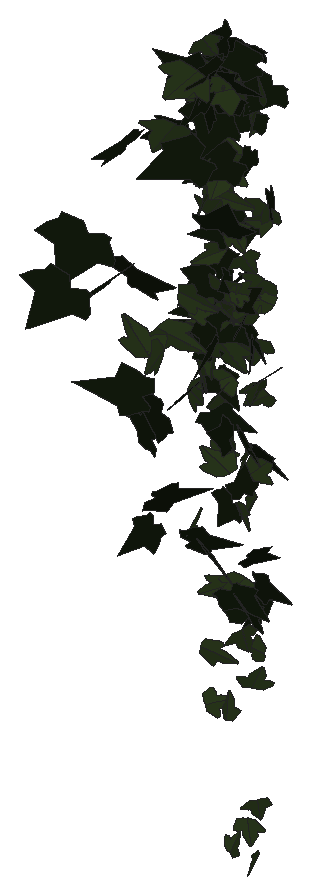
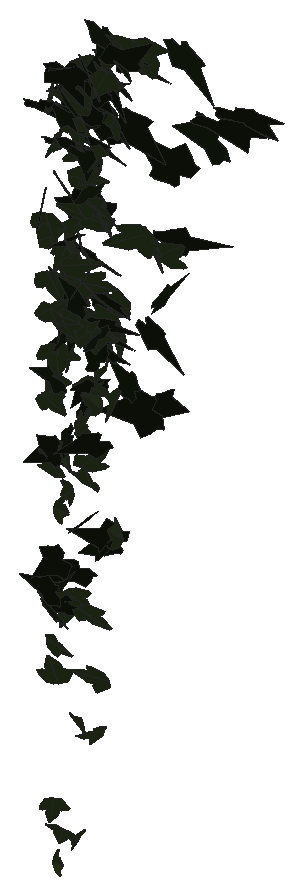
# SketchUp Ruby script. Lengths in inches.
U = 1.inch
M = Sketchup.active_model
def pt(a) = Geom::Point3d.new(a.map { |v| v * U })
def face(e, loops, mat)
  f = e.add_face(loops[0].map { |a| pt(a) })
  loops[1..].each { |l| e.add_face(l.map { |a| pt(a) }).erase! }
  f.material = f.back_material = mat if mat
  f
end
# faces: each face lists its corners as indices into pts; further lists are holes
def faces(e, pts, list, mat = nil) = list.each { |f| face(e, (f[0].is_a?(Array) ? f : [f]).map { |l| l.map { |i| pts[i] } }, mat) }
# xy, xz, yz: faces in a plane at the given z, y or x. An outline is a flat list of corners, or four numbers for a rectangle; further outlines are holes
def ring(l) = l.size == 4 ? [[l[0], l[1]], [l[2], l[1]], [l[2], l[3]], [l[0], l[3]]] : l.each_slice(2).to_a
def flat(e, list, mat, &to3) = list.each { |f| face(e, (f[0].is_a?(Array) ? f : [f]).map { |l| ring(l).map { |u, v| to3.(u, v) } }, mat) }
def xy(e, z, list, mat = nil) = flat(e, list, mat) { |x, y| [x, y, z] }
def xz(e, y, list, mat = nil) = flat(e, list, mat) { |x, z| [x, y, z] }
def yz(e, x, list, mat = nil) = flat(e, list, mat) { |y, z| [x, y, z] }
def lines(e, pts, list) = list.each { |a, b| e.add_line(pt(pts[a]), pt(pts[b])) }
# prism: a flat outline (further loops are holes) pulled along v
def prism(e, loops, v, mat = nil)
  f = face(e, loops, mat); d = Geom::Vector3d.new(v.map { |x| x * U })
  f.pushpull(f.normal.samedirection?(d) ? d.length : -d.length)
end
def box(e, o, s, mat = nil) = prism(e, [[o, [o[0] + s[0], o[1], o[2]], [o[0] + s[0], o[1] + s[1], o[2]], [o[0], o[1] + s[1], o[2]]]], [0, 0, s[2]], mat)
def at(x, y, z, deg = 0) = Geom::Transformation.translation(pt([x, y, z])) * Geom::Transformation.rotation(ORIGIN, Z_AXIS, deg.degrees)
def axes(o, x, y, z) = Geom::Transformation.new([*x, 0, *y, 0, *z, 0, *pt(o).to_a, 1])
def part(name) = M.definitions.add(name)
# library, detail: a bought-in or finely detailed component or shape, given as its bounding box
def library(name, o, s) = part(name).tap { |d| box(d.entities, o, s) }
def detail(e, o, s) = box(e.add_group.entities, o, s)
def put(e, d, t, mat = nil) = e.add_instance(d, t).tap { |i| i.material = mat if mat }
def group(e, t, mat = nil) = e.add_group.tap { |g| g.transformation = t; g.material = mat if mat }.entities
root = M.entities
M.materials.add("1026 AP 7946 SUNNY SIDE UP").color = [254, 231, 186]
M.materials.add("efeu1").color = [18, 25, 13]
M.materials.add("efeu2").color = [43, 57, 29]
c1 = part("ivyleaf_9")
p = [[1.54,2.16,1.25],[1.36,2.04,1.19],[-0.21,0.99,0.68],[-0.71,1.11,0.82],[-0.85,0.86,0.67],[-0.8,0.17,0.21],
  [-0.9,-0.01,0.1],[-0.67,-0.16,-0.02],[-0.08,-0.08,-0.05],[-0.03,-0.6,-0.4],[0.65,-0.88,-0.66],[0.83,-0.6,-0.49],
  [1.29,-0.42,-0.43],[1.8125,-0.07,-0.26],[1.21,0.44,0.15]]
faces(c1.entities,p,[[0,1,2,3,4,5,6,7,8,9,10,11,12,13,14]],"efeu1")
c2 = part("ivyleaf_10")
p = [[0,0.5,-0.03],[-0.0625,2.02,-0.43],[-0.19,2.01,-0.46],[-0.54,1.05,-0.29],[-0.52,0.625,-0.18],[-0.83,0.76,-0.28],
  [-1.16,0.64,-0.33],[-1.15,0.33,-0.24],[-0.77,-0.39,0.02],[-0.3,-0.51,0.16],[0.04,-0.48,0.23],[-0.02,2.01,-0.4375],
  [-0.06,2.01,-0.43],[0.04,-0.49,0.23],[0.67,-0.49,0.14],[1.38,0.36,-0.2],[1.375,0.51,-0.24],[0.81,0.65,-0.19],
  [0.62,0.59,-0.15],[0.6,1.09,-0.28],[0.5,1.23,-0.31]]
faces(c2.entities,p,[[0,1,2,3,4,5,6,7,8,9,10],[11,12,0,13,14,15,16,17,18,19,20]],"efeu2")
put(root,c1,axes([97.74,206.36,264.18],[-0.57261,-0.15899,0.00661],[0.01155,-0.03369,-0.3981],[0.27002,-0.33573,0.03104]),"1026 AP 7946 SUNNY SIDE UP")
put(root,c1,axes([97.83,206.99,263.79],[-0.11865,0.31649,-0.13339],[-0.03463,0.12729,0.34869],[0.57896,0.07247,-0.00648]),"1026 AP 7946 SUNNY SIDE UP")
put(root,c1,axes([97.2,207.625,264.69],[-0.57225,-0.19595,-0.07876],[0.1339,0.00504,-0.41571],[0.32748,-0.34446,0.03235]),"1026 AP 7946 SUNNY SIDE UP")
put(root,c1,axes([98.54,207.72,261.34],[-0.28709,-0.00794,0.3068],[-0.47432,-0.07037,-0.17955],[0.10962,-0.32532,0.02659]),"1026 AP 7946 SUNNY SIDE UP")
put(root,c1,axes([98.41,208.22,260.1],[0.00994,-0.29617,0.10479],[0.00181,0.10178,0.31854],[-0.53159,-0.00519,0.00305]),"1026 AP 7946 SUNNY SIDE UP")
put(root,c1,axes([97.77,208.36,263.6],[0.05912,-0.09662,0.33615],[0.41432,-0.20559,-0.09919],[0.37633,0.24152,0.0564]),"1026 AP 7946 SUNNY SIDE UP")
put(root,c1,axes([98.23,208.49,257.8],[-0.01657,-0.03364,-0.32985],[0.19296,-0.2867,0.0257],[-0.48867,-0.11207,0.02133]),"1026 AP 7946 SUNNY SIDE UP")
put(root,c1,axes([97.62,208.38,266.64],[-0.23235,0.33578,-0.00813],[-0.01483,-0.01648,-0.38812],[-0.57017,-0.1364,0.01341]),"1026 AP 7946 SUNNY SIDE UP")
put(root,c2,axes([98.32,208.6,261.89],[0.27853,-0.2642,-0.07494],[-0.07251,0.05179,-0.3321],[0.45679,0.16932,-0.00702]),"1026 AP 7946 SUNNY SIDE UP")
put(root,c2,axes([97.84,208.8,261.74],[0.42097,0.06657,0.18504],[-0.29585,-0.00962,0.2729],[0.10235,-0.30163,0.02772]),"1026 AP 7946 SUNNY SIDE UP")
put(root,c1,axes([98.88,209.1875,266.44],[-0.59553,-0.0337,0.08502],[-0.12333,-0.06727,-0.37301],[0.08025,-0.35345,0.05773]),"1026 AP 7946 SUNNY SIDE UP")
put(root,c2,axes([98.22,209.02,262.17],[-0.23906,-0.09754,-0.28056],[0.42891,0.07804,-0.17622],[0.19861,-0.28593,0.04286]),"1026 AP 7946 SUNNY SIDE UP")
put(root,c2,axes([98.18,209.22,266.87],[-0.36364,-0.18696,0.13786],[-0.13468,-0.10778,-0.30458],[0.36358,-0.22691,0.02506]),"1026 AP 7946 SUNNY SIDE UP")
put(root,c1,axes([97.92,209.15,260.09],[0.02255,-0.02389,-0.34779],[-0.55102,-0.02407,-0.01266],[-0.03928,0.32393,-0.02202]),"1026 AP 7946 SUNNY SIDE UP")
put(root,c1,axes([97.91,209.13,258.08],[0.04211,0.20914,-0.26445],[-0.00016,0.25047,0.22804],[0.55297,-0.01585,0.0202]),"1026 AP 7946 SUNNY SIDE UP")
put(root,c2,axes([97.86,210.24,267.56],[0.52572,-0.05732,-0.1389],[-0.22518,-0.01183,-0.33548],[0.08194,0.33528,-0.03076]),"1026 AP 7946 SUNNY SIDE UP")
put(root,c1,axes([98.32,210.45,261.27],[-0.2559,0.10294,-0.21454],[0.25125,-0.13866,-0.19608],[-0.29101,-0.21023,0.01936]),"1026 AP 7946 SUNNY SIDE UP")
put(root,c1,axes([98.07,210.53,267.0625],[-0.40271,0.1267,-0.20041],[0.24447,-0.1275,-0.28704],[-0.29877,-0.27511,0.03526]),"1026 AP 7946 SUNNY SIDE UP")
put(root,c1,axes([98.24,210.32,267.7],[-0.19473,0.30654,0.05328],[-0.06802,0.03373,-0.34887],[-0.52171,-0.11882,0.02559]),"1026 AP 7946 SUNNY SIDE UP")
put(root,c1,axes([98.19,210.68,266.55],[-0.27394,-0.27734,0.04395],[0.01113,-0.05522,-0.34245],[0.47673,-0.15808,0.03325]),"1026 AP 7946 SUNNY SIDE UP")
put(root,c1,axes([97.57,210.64,267.34],[0.06166,0.02742,0.27711],[-0.42307,-0.07047,0.04451],[0.12535,-0.25133,0.01393]),"1026 AP 7946 SUNNY SIDE UP")
put(root,c1,axes([97.51,210.6,265.94],[0.0325,0.11967,-0.31584],[-0.40785,-0.19071,-0.10165],[-0.35832,0.22794,0.08705]),"1026 AP 7946 SUNNY SIDE UP")
put(root,c1,axes([97.23,210.5625,259.46],[0.08556,0.22977,0.0797],[-0.03764,-0.06826,0.25078],[0.40672,-0.05465,0.00644]),"1026 AP 7946 SUNNY SIDE UP")
put(root,c1,axes([98.05,210.52,266.88],[0.09166,-0.03664,-0.34822],[-0.55011,0.03688,-0.06161],[0.07227,0.32717,-0.02737]),"1026 AP 7946 SUNNY SIDE UP")
put(root,c1,axes([98.15,210.59,266.2],[-0.2466,0.28893,0.03803],[-0.05451,0.01933,-0.34529],[-0.4904,-0.14744,0.01926]),"1026 AP 7946 SUNNY SIDE UP")
put(root,c2,axes([98.3,210.78,267.125],[0.3436,-0.01208,-0.24927],[-0.39361,-0.04066,-0.21425],[-0.03877,0.30571,-0.034]),"1026 AP 7946 SUNNY SIDE UP")
put(root,c2,axes([97.6875,210.79,260.38],[-0.14335,0.16252,-0.14526],[0.08778,-0.12817,-0.19753],[-0.35089,-0.09845,0.00993]),"1026 AP 7946 SUNNY SIDE UP")
put(root,c1,axes([97.98,210.53,267.06],[0.04189,0.05592,0.34926],[0.19375,0.30486,-0.06108],[-0.52611,0.11672,0.00531]),"1026 AP 7946 SUNNY SIDE UP")
put(root,c1,axes([98.4,210.91,265.43],[-0.5274,0.01258,0.02252],[-0.03777,-0.03758,-0.33087],[-0.01687,-0.30911,0.03675]),"1026 AP 7946 SUNNY SIDE UP")
put(root,c1,axes([98.24,211.03,258.75],[-0.05289,0.00628,0.28],[-0.19704,-0.24335,-0.01161],[0.37929,-0.12555,0.03301]),"1026 AP 7946 SUNNY SIDE UP")
put(root,c2,axes([98.36,210.82,261.02],[-0.38061,-0.08114,-0.12402],[0.19478,0.0192,-0.2542],[0.13786,-0.25115,0.01674]),"1026 AP 7946 SUNNY SIDE UP")
put(root,c2,axes([98.125,210.98,265.12],[0.34628,0.19807,-0.11587],[-0.09819,-0.0987,-0.30425],[-0.37256,0.21012,-0.02751]),"1026 AP 7946 SUNNY SIDE UP")
put(root,c2,axes([97.5625,211.09,267.14],[-0.01804,-0.04519,-0.29112],[0.31158,-0.20342,0.02573],[-0.3478,-0.17989,0.03815]),"1026 AP 7946 SUNNY SIDE UP")
put(root,c1,axes([98,211.01,263.67],[0.4799,0.04574,0.1037],[-0.16985,0.01988,0.30473],[0.06234,-0.29798,0.03197]),"1026 AP 7946 SUNNY SIDE UP")
put(root,c2,axes([97.33,210.89,260.93],[-0.27622,0.1351,0.10261],[-0.14652,0.04264,-0.22477],[-0.23799,-0.18306,0.01929]),"1026 AP 7946 SUNNY SIDE UP")
put(root,c1,axes([98.1875,211.05,266.78],[0.04129,0.10514,-0.23875],[-0.08837,-0.21825,-0.11857],[-0.41124,0.05746,0.00151]),"1026 AP 7946 SUNNY SIDE UP")
put(root,c2,axes([97.11,211.05,261.73],[0.00993,0.00527,0.26951],[0.42354,0.03325,-0.00649],[-0.05664,0.24953,-0.00128]),"1026 AP 7946 SUNNY SIDE UP")
put(root,c1,axes([97.46,211.21,255.86],[0.27721,-0.17436,0.024],[0.01098,-0.02772,-0.25569],[0.29873,0.16282,-0.01288]),"1026 AP 7946 SUNNY SIDE UP")
put(root,c1,axes([98.0625,211.37,261.22],[-0.1776,-0.21685,0.09937],[0.01531,-0.10812,-0.25337],[0.40203,-0.09168,0.05355]),"1026 AP 7946 SUNNY SIDE UP")
put(root,c1,axes([97.78,211.2,261.01],[-0.17558,-0.06474,-0.21683],[-0.33041,-0.0595,0.12648],[-0.14187,0.21871,-0.02623]),"1026 AP 7946 SUNNY SIDE UP")
put(root,c1,axes([97.24,211.11,255.95],[0.16281,0.01928,0.24539],[0.3754,0.00007,-0.10696],[-0.01219,0.25963,-0.01666]),"1026 AP 7946 SUNNY SIDE UP")
put(root,c1,axes([97.65,211.15,260.57],[-0.118,0.09448,0.2043],[-0.22868,0.13428,-0.12264],[-0.27752,-0.15083,0.01419]),"1026 AP 7946 SUNNY SIDE UP")
put(root,c2,axes([97.25,211.09,259.49],[-0.06479,0.1857,0.19848],[-0.10528,0.17314,-0.19956],[-0.42984,-0.0704,0.01896]),"1026 AP 7946 SUNNY SIDE UP")
put(root,c2,axes([97.14,211.15,256.13],[0.11146,-0.16396,0.19281],[-0.10119,0.1769,0.18488],[-0.37907,-0.09543,0.00734]),"1026 AP 7946 SUNNY SIDE UP")
put(root,c2,axes([98.4375,211.24,254.13],[-0.15022,-0.23114,-0.09448],[0.08508,0.07514,-0.25639],[0.38087,-0.10795,0.02]),"1026 AP 7946 SUNNY SIDE UP")
put(root,c1,axes([98.2,211.23,255.03],[-0.02195,-0.07115,-0.24722],[0.15638,0.21134,-0.07258],[0.37758,-0.09167,0.01569]),"1026 AP 7946 SUNNY SIDE UP")
put(root,c2,axes([97.53,211.33,263.73],[-0.35968,0.05025,0.11447],[0.18472,0.00098,0.23179],[0.07548,0.23704,-0.02177]),"1026 AP 7946 SUNNY SIDE UP")
put(root,c2,axes([97.7,211.37,261.04],[-0.02678,0.03351,0.23081],[-0.31788,-0.11218,0.00244],[0.18865,-0.18427,0.03688]),"1026 AP 7946 SUNNY SIDE UP")
put(root,c2,axes([98.05,211.34,261.18],[0.12188,0.20803,-0.06657],[-0.0288,-0.06279,-0.23644],[-0.36881,0.07365,-0.00354]),"1026 AP 7946 SUNNY SIDE UP")
put(root,c2,axes([97.84,211.32,261.98],[-0.30306,0.01026,0.16283],[0.25841,0.01977,0.1903],[-0.00857,0.23361,-0.01997]),"1026 AP 7946 SUNNY SIDE UP")
put(root,c1,axes([97.62,211.21,266.95],[0.34735,0.05393,0.18451],[0.29276,0.01525,-0.22503],[-0.087,0.26664,-0.02056]),"1026 AP 7946 SUNNY SIDE UP")
put(root,c2,axes([98.28,211.39,256.98],[-0.1745,0.11775,-0.12685],[0.10847,-0.10276,-0.16796],[-0.264,-0.12005,0.01483]),"1026 AP 7946 SUNNY SIDE UP")
put(root,c1,axes([97.47,211.45,262.07],[-0.44924,-0.0264,-0.02736],[0.04764,-0.02916,-0.28311],[0.03962,-0.26423,0.03021]),"1026 AP 7946 SUNNY SIDE UP")
put(root,c2,axes([97.82,211.38,257.77],[0.17276,0.19348,0.13707],[-0.12418,-0.10302,0.23208],[0.37127,-0.12448,0.01385]),"1026 AP 7946 SUNNY SIDE UP")
put(root,c2,axes([97.16,211.36,266.34],[-0.31264,0.13083,-0.08864],[0.09833,-0.06393,-0.24203],[-0.24541,-0.19228,0.01594]),"1026 AP 7946 SUNNY SIDE UP")
put(root,c2,axes([98.02,211.375,258.5],[-0.26648,0.1249,0.05204],[0.07414,-0.02046,0.21416],[0.21405,0.16258,-0.00939]),"1026 AP 7946 SUNNY SIDE UP")
put(root,c1,axes([97.92,211.54,262.13],[0.11581,-0.14783,-0.1752],[0.17868,-0.12645,0.16951],[-0.32622,-0.12174,0.03065]),"1026 AP 7946 SUNNY SIDE UP")
put(root,c2,axes([98.14,211.28,263.54],[0.07704,0.22951,0.09905],[0.01981,0.08893,-0.24916],[-0.41773,0.04654,0.00645]),"1026 AP 7946 SUNNY SIDE UP")
put(root,c2,axes([97.26,211.28,261.4],[0.0644,0.03555,0.27371],[0.34022,0.15805,-0.05326],[-0.2749,0.20393,-0.0018]),"1026 AP 7946 SUNNY SIDE UP")
put(root,c1,axes([97.52,211.53,261.38],[-0.33434,-0.04721,0.15768],[-0.22963,-0.06507,-0.21599],[0.12934,-0.23756,0.02413]),"1026 AP 7946 SUNNY SIDE UP")
put(root,c2,axes([97.61,211.32,259.25],[0.07104,-0.18576,0.15118],[-0.00972,0.14504,0.20464],[-0.39849,-0.03666,0.02196]),"1026 AP 7946 SUNNY SIDE UP")
put(root,c2,axes([97.35,211.51,264.16],[0.1883,-0.25191,0.06776],[0.02774,-0.06549,-0.29535],[0.44144,0.11157,-0.01035]),"1026 AP 7946 SUNNY SIDE UP")
put(root,c2,axes([97.77,211.5,259.81],[0.21637,0.05238,-0.19672],[-0.27439,-0.08975,-0.14813],[-0.17504,0.20544,-0.01095]),"1026 AP 7946 SUNNY SIDE UP")
put(root,c1,axes([98.42,211.32,257.45],[-0.30439,0.10202,-0.05147],[-0.06236,0.03516,0.22098],[0.18204,0.18264,-0.01036]),"1026 AP 7946 SUNNY SIDE UP")
put(root,c1,axes([98.59,211.53,254.4],[0.0718,-0.21808,0.04231],[0.00065,0.04319,0.23825],[-0.37711,-0.04145,0.00846]),"1026 AP 7946 SUNNY SIDE UP")
put(root,c2,axes([98.27,211.29,262.1],[0.05294,0.07266,0.22732],[0.0632,0.20877,-0.07979],[-0.37415,0.04555,0.01869]),"1026 AP 7946 SUNNY SIDE UP")
put(root,c1,axes([98.07,211.49,261.75],[-0.11481,0.0702,0.22043],[0.25111,-0.14195,0.10232],[0.26875,0.16262,-0.00143]),"1026 AP 7946 SUNNY SIDE UP")
put(root,c2,axes([97.5,211.33,260],[0.0122,0.15486,-0.19105],[0.01374,0.18029,0.16848],[0.40345,-0.01082,0.00004]),"1026 AP 7946 SUNNY SIDE UP")
put(root,c1,axes([97.59,211.48,259.86],[0.01616,-0.19043,-0.1791],[-0.0197,0.16442,-0.20181],[0.42706,0.01479,-0.00253]),"1026 AP 7946 SUNNY SIDE UP")
put(root,c2,axes([98.33,211.45,262.88],[-0.17548,-0.18117,-0.12736],[0.11953,0.09381,-0.22158],[0.34565,-0.12442,0.01197]),"1026 AP 7946 SUNNY SIDE UP")
put(root,c2,axes([97.67,211.57,261.29],[-0.29394,0.06963,0.14956],[0.21934,-0.05067,0.19909],[0.14617,0.21605,0.00199]),"1026 AP 7946 SUNNY SIDE UP")
put(root,c1,axes([97.28,211.68,261.15],[0.10496,-0.21477,0.14519],[0.05546,-0.1346,-0.24109],[0.43018,0.06975,-0.00434]),"1026 AP 7946 SUNNY SIDE UP")
put(root,c2,axes([97.59,211.55,261.09],[-0.35864,-0.0561,0.12544],[-0.1806,-0.05605,-0.23343],[0.12849,-0.23536,0.02203]),"1026 AP 7946 SUNNY SIDE UP")
put(root,c1,axes([98.36,211.66,260.8],[-0.0456,0.00496,-0.23103],[0.3,-0.12446,-0.02834],[-0.21057,-0.1784,0.00965]),"1026 AP 7946 SUNNY SIDE UP")
put(root,c1,axes([97.22,211.72,260.66],[0.09575,-0.15393,0.20709],[0.11065,-0.18925,-0.17162],[0.38356,0.09302,-0.00219]),"1026 AP 7946 SUNNY SIDE UP")
put(root,c2,axes([97.61,211.62,264.33],[-0.19597,0.0003,0.22574],[-0.34799,-0.05642,-0.12086],[0.08378,-0.23367,0.02603]),"1026 AP 7946 SUNNY SIDE UP")
put(root,c1,axes([98.17,211.42,261.09],[-0.10155,0.04078,-0.26841],[-0.29527,0.18157,0.07822],[0.29166,0.19801,-0.01427]),"1026 AP 7946 SUNNY SIDE UP")
put(root,c2,axes([97.46,211.59,263.98],[-0.05208,0.02119,0.29585],[0.45024,0.08198,0.02597],[-0.13491,0.2654,-0.02756]),"1026 AP 7946 SUNNY SIDE UP")
put(root,c2,axes([98.1875,211.75,261.4],[-0.14383,-0.09885,0.18719],[-0.1415,-0.15688,-0.13936],[0.31231,-0.1166,0.02307]),"1026 AP 7946 SUNNY SIDE UP")
put(root,c1,axes([97.75,211.66,263.18],[-0.33186,0.09772,0.08763],[-0.14091,0.0131,-0.23241],[-0.16241,-0.21105,0.02257]),"1026 AP 7946 SUNNY SIDE UP")
put(root,c2,axes([98.15,211.5,260.47],[-0.08636,0.11086,0.2022],[-0.15763,0.16305,-0.12795],[-0.33436,-0.1055,0.0081]),"1026 AP 7946 SUNNY SIDE UP")
put(root,c2,axes([97.17,211.59,267.53],[-0.17739,-0.18003,-0.13344],[0.13799,0.09356,-0.22051],[0.34272,-0.13085,0.01972]),"1026 AP 7946 SUNNY SIDE UP")
put(root,c1,axes([98.27,211.81,267.3],[-0.25582,-0.02335,0.21927],[-0.328,-0.07349,-0.16196],[0.12342,-0.24369,0.02409]),"1026 AP 7946 SUNNY SIDE UP")
put(root,c2,axes([97.4,211.83,262.54],[0.1269,0.07699,-0.25136],[-0.27391,-0.17194,-0.11727],[-0.3198,0.17782,0.0007]),"1026 AP 7946 SUNNY SIDE UP")
put(root,c1,axes([98.0625,211.68,258.5],[0.27509,-0.13401,-0.11246],[-0.15453,0.05152,-0.22372],[0.24211,0.18514,-0.01501]),"1026 AP 7946 SUNNY SIDE UP")
put(root,c2,axes([97.76,211.68,261.45],[-0.2507,-0.19578,-0.08763],[0.13743,0.03691,-0.25845],[0.3312,-0.16351,0.04091]),"1026 AP 7946 SUNNY SIDE UP")
put(root,c2,axes([97.89,211.5625,248.71],[0.06942,0.07772,-0.18665],[0.02957,0.1836,0.08672],[0.30921,-0.03501,0.03361]),"1026 AP 7946 SUNNY SIDE UP")
put(root,c2,axes([98.18,211.76,258.14],[0.09264,-0.20786,0.02191],[0.00468,-0.02323,-0.23037],[0.35501,0.05455,-0.00268]),"1026 AP 7946 SUNNY SIDE UP")
put(root,c2,axes([97.73,211.83,265],[0.01748,0.02752,0.23904],[-0.26423,-0.16001,0.02661],[0.2749,-0.15556,0.01038]),"1026 AP 7946 SUNNY SIDE UP")
put(root,c2,axes([98.41,211.77,259.75],[-0.08749,-0.23047,0.02394],[-0.0006,-0.02591,-0.25313],[0.3936,-0.05127,0.00494]),"1026 AP 7946 SUNNY SIDE UP")
put(root,c1,axes([97.59,211.94,256.61],[-0.09557,-0.18183,0.15477],[-0.05284,-0.14795,-0.198],[0.36813,-0.06844,0.01176]),"1026 AP 7946 SUNNY SIDE UP")
put(root,c2,axes([98.54,211.76,262.25],[-0.3376,-0.05316,0.10758],[-0.15524,-0.0478,-0.21998],[0.11638,-0.21795,0.01863]),"1026 AP 7946 SUNNY SIDE UP")
put(root,c1,axes([97.73,211.69,262.4],[-0.24348,0.15689,0.09729],[-0.12124,0.05478,-0.22628],[-0.28101,-0.15957,0.01333]),"1026 AP 7946 SUNNY SIDE UP")
put(root,c1,axes([97.7,211.7,261.85],[0.08145,0.23853,0.054],[-0.04236,-0.04316,0.25934],[0.41064,-0.05177,0.01604]),"1026 AP 7946 SUNNY SIDE UP")
put(root,c1,axes([98,211.87,261.04],[0.1958,-0.22739,0.00991],[-0.01599,-0.01846,-0.27264],[0.38623,0.11451,-0.01631]),"1026 AP 7946 SUNNY SIDE UP")
put(root,c1,axes([98.39,211.65,259.79],[-0.03945,0.20029,-0.07468],[-0.00997,0.07217,0.21685],[0.36137,0.02385,-0.00217]),"1026 AP 7946 SUNNY SIDE UP")
put(root,c1,axes([98.17,211.74,254.23],[-0.33947,-0.05695,0.10896],[0.15395,0.04377,0.22971],[-0.11022,0.23653,-0.01476]),"1026 AP 7946 SUNNY SIDE UP")
put(root,c1,axes([97.66,211.69,267.7],[-0.08187,-0.01029,-0.28258],[-0.42174,0.09253,0.04605],[0.15168,0.25172,-0.02449]),"1026 AP 7946 SUNNY SIDE UP")
put(root,c2,axes([98.12,211.99,256.83],[0.04934,-0.11847,0.19292],[0.08633,-0.17978,-0.12725],[0.33849,0.06312,0.00433]),"1026 AP 7946 SUNNY SIDE UP")
put(root,c2,axes([98.28,211.84,252.61],[-0.25048,-0.15897,0.04346],[0.03292,0.03991,0.23167],[-0.25688,0.16012,-0.01269]),"1026 AP 7946 SUNNY SIDE UP")
put(root,c1,axes([97.96,211.98,263.45],[-0.09016,-0.21653,0.039],[-0.00421,-0.03978,-0.23913],[0.37354,-0.05271,0.00672]),"1026 AP 7946 SUNNY SIDE UP")
put(root,c2,axes([97.0625,211.86,253],[-0.06039,-0.01539,-0.2387],[0.3587,-0.04594,-0.03609],[-0.06753,-0.23024,0.02175]),"1026 AP 7946 SUNNY SIDE UP")
put(root,c2,axes([98.28,211.86,257.64],[0.30501,-0.08918,-0.119],[0.18364,-0.02821,0.21328],[-0.1551,-0.20877,0.01851]),"1026 AP 7946 SUNNY SIDE UP")
put(root,c1,axes([97.18,212.04,266.53],[-0.06689,-0.19302,0.16073],[0.08128,-0.16277,-0.19254],[0.3828,0.00083,0.06896]),"1026 AP 7946 SUNNY SIDE UP")
put(root,c2,axes([97.84,211.93,254.84],[0.27751,0.08845,-0.14806],[-0.19211,-0.07753,-0.20347],[-0.18402,0.21433,-0.01086]),"1026 AP 7946 SUNNY SIDE UP")
put(root,c2,axes([97.9,211.91,263.38],[0.12612,-0.20956,0.02513],[0.00281,-0.0272,-0.23827],[0.35849,0.07394,-0.00697]),"1026 AP 7946 SUNNY SIDE UP")
put(root,c1,axes([98.29,211.85,258.16],[0.36675,-0.05403,0.0293],[0.0369,-0.02821,-0.23765],[0.09654,0.21603,-0.02045]),"1026 AP 7946 SUNNY SIDE UP")
put(root,c2,axes([98.26,211.91,260.63],[-0.33398,-0.15579,0.02291],[-0.00997,-0.0302,-0.26824],[0.26726,-0.19582,0.01862]),"1026 AP 7946 SUNNY SIDE UP")
put(root,c1,axes([97.24,211.76,258.71],[0.11227,-0.04977,-0.26525],[0.05792,0.26584,-0.0409],[0.40783,-0.02405,0.07883]),"1026 AP 7946 SUNNY SIDE UP")
put(root,c2,axes([98.43,211.93,266.57],[-0.20819,0.20561,0.07455],[0.07474,-0.05162,0.25531],[0.35937,0.12985,-0.00991]),"1026 AP 7946 SUNNY SIDE UP")
put(root,c2,axes([98.4,211.87,253.42],[0.00106,0.0415,0.21454],[-0.33306,0.01122,-0.00153],[-0.01777,-0.20771,0.04152]),"1026 AP 7946 SUNNY SIDE UP")
put(root,c2,axes([97.4,211.96,254.58],[0.25664,-0.00526,-0.1805],[-0.27484,-0.02229,-0.16721],[-0.02004,0.23839,-0.01821]),"1026 AP 7946 SUNNY SIDE UP")
put(root,c1,axes([97.55,211.76,265.67],[0.03388,0.21831,0.07441],[-0.00114,0.06697,-0.23365],[-0.38748,0.01889,0.0072]),"1026 AP 7946 SUNNY SIDE UP")
put(root,c2,axes([98.44,211.97,259.43],[-0.19878,-0.06572,0.14812],[-0.17949,-0.0928,-0.14341],[0.18995,-0.15646,0.0195]),"1026 AP 7946 SUNNY SIDE UP")
put(root,c1,axes([97.99,211.9,267.59],[0.16601,0.13135,-0.1967],[-0.26599,-0.10725,-0.17129],[-0.27941,0.18014,0.04619]),"1026 AP 7946 SUNNY SIDE UP")
put(root,c2,axes([97.68,212.1,262.97],[0.01603,0.05119,0.26724],[-0.17935,-0.23303,0.05069],[0.37459,-0.11376,0.01283]),"1026 AP 7946 SUNNY SIDE UP")
put(root,c2,axes([97.56,211.89,251.63],[0.27124,-0.10136,0.09786],[-0.11251,0.06605,0.2056],[-0.18795,-0.18582,0.01816]),"1026 AP 7946 SUNNY SIDE UP")
put(root,c2,axes([97.36,211.97,265.14],[-0.0087,0.23556,0.06939],[-0.00056,-0.06177,0.25138],[0.41338,0.00488,0.0018]),"1026 AP 7946 SUNNY SIDE UP")
put(root,c2,axes([97.99,211.96,266.34],[-0.13613,0.23583,-0.05798],[0.00804,-0.05874,-0.26707],[-0.41188,-0.07909,0.01395]),"1026 AP 7946 SUNNY SIDE UP")
put(root,c1,axes([98.05,212.09,265.93],[-0.40124,-0.08143,0.02693],[-0.0238,-0.03911,-0.26595],[0.14325,-0.23458,0.03123]),"1026 AP 7946 SUNNY SIDE UP")
put(root,c2,axes([98.39,212.09,261.57],[0.04024,0.16602,0.21438],[-0.09437,-0.19911,0.17086],[0.40662,-0.06264,0.01844]),"1026 AP 7946 SUNNY SIDE UP")
put(root,c2,axes([98.08,211.93,261.35],[0.23624,0.02336,0.20336],[-0.32437,0.0156,0.14827],[0.00195,-0.23471,0.02677]),"1026 AP 7946 SUNNY SIDE UP")
put(root,c2,axes([97.32,211.94,257.73],[0.34096,-0.05968,0.01123],[-0.00696,0.02605,0.23053],[-0.09524,-0.21556,0.02337]),"1026 AP 7946 SUNNY SIDE UP")
put(root,c1,axes([97.97,212.09,264.9375],[-0.24822,0.01168,-0.17358],[0.25552,-0.07313,-0.15185],[-0.10486,-0.20584,0.04086]),"1026 AP 7946 SUNNY SIDE UP")
put(root,c1,axes([97.95,212.02,266.73],[-0.19647,0.1991,-0.12994],[0.07413,-0.11753,-0.24737],[-0.39118,-0.12227,0.01839]),"1026 AP 7946 SUNNY SIDE UP")
put(root,c1,axes([98.47,212.14,266.7],[-0.39526,-0.12405,-0.00512],[0.0275,-0.02372,-0.28112],[0.20884,-0.23166,0.02733]),"1026 AP 7946 SUNNY SIDE UP")
put(root,c1,axes([98.42,212.07,254.51],[-0.3113,0.09921,-0.11848],[0.14283,-0.07523,-0.22728],[-0.19224,-0.21655,0.02299]),"1026 AP 7946 SUNNY SIDE UP")
put(root,c2,axes([98.37,212.18,263.47],[-0.02423,-0.03844,-0.24668],[-0.19805,-0.19824,0.04047],[-0.34258,0.11732,-0.00595]),"1026 AP 7946 SUNNY SIDE UP")
put(root,c2,axes([97.4375,212,266.96],[-0.06197,0.00602,0.28773],[0.42689,0.06717,0.03837],[-0.10333,0.27392,-0.01404]),"1026 AP 7946 SUNNY SIDE UP")
put(root,c2,axes([98.04,212.16,248.28],[0.08925,-0.09381,0.17811],[0.11524,-0.15749,-0.1134],[0.28781,0.09215,-0.00982]),"1026 AP 7946 SUNNY SIDE UP")
put(root,c1,axes([96.86,212.09,266.81],[0.0493,-0.06356,-0.27271],[0.41774,0.06375,0.01704],[0.09092,-0.25846,0.06957]),"1026 AP 7946 SUNNY SIDE UP")
put(root,c2,axes([98.43,212.02,263.83],[-0.36982,0.0179,0.10011],[-0.16096,-0.02721,-0.23187],[-0.00952,-0.23542,0.03106]),"1026 AP 7946 SUNNY SIDE UP")
put(root,c1,axes([97.11,212.21,264.92],[-0.03351,-0.19444,0.15095],[0.07302,-0.14871,-0.19575],[0.37687,0.01153,0.05135]),"1026 AP 7946 SUNNY SIDE UP")
put(root,c2,axes([97.92,212.07,249.08],[0.30073,0.03219,0.06012],[0.09512,-0.01074,-0.19882],[-0.04338,0.19962,-0.01919]),"1026 AP 7946 SUNNY SIDE UP")
put(root,c2,axes([97.42,212.14,259.09],[-0.07024,0.17046,0.15029],[0.05259,-0.14103,0.1807],[0.34785,0.05575,0.00303]),"1026 AP 7946 SUNNY SIDE UP")
put(root,c1,axes([98.17,212.09,254.85],[0.16888,-0.05705,-0.21705],[0.33657,0.07184,0.09293],[0.06465,-0.225,0.08317]),"1026 AP 7946 SUNNY SIDE UP")
put(root,c2,axes([98.11,212.16,265.85],[0.03018,0.13631,-0.17682],[-0.03946,-0.16532,-0.14947],[-0.36373,0.02925,0.00154]),"1026 AP 7946 SUNNY SIDE UP")
put(root,c2,axes([97.62,212.02,266.42],[-0.35121,0.08849,0.09341],[-0.15203,0.0081,-0.23919],[-0.14428,-0.22395,0.02464]),"1026 AP 7946 SUNNY SIDE UP")
put(root,c1,axes([98.51,212.15,263.8],[-0.06995,0.11055,0.22067],[-0.12605,-0.20324,0.09868],[0.37423,-0.04779,0.07449]),"1026 AP 7946 SUNNY SIDE UP")
put(root,c2,axes([97.06,211.91,251.72],[0.10295,-0.03126,-0.22096],[0.1991,0.18716,0.01282],[0.27628,-0.12323,0.0731]),"1026 AP 7946 SUNNY SIDE UP")
put(root,c1,axes([98.13,211.88,255.53],[0.17844,0.15788,0.15748],[0.16662,0.11026,-0.19888],[-0.30159,0.15432,-0.0167]),"1026 AP 7946 SUNNY SIDE UP")
put(root,c1,axes([97.82,212.16,267.1],[-0.33364,0.09477,-0.1548],[0.19699,-0.09244,-0.23305],[-0.2199,-0.2266,0.02609]),"1026 AP 7946 SUNNY SIDE UP")
put(root,c2,axes([98.19,212.07,249.67],[-0.18612,-0.16466,-0.03355],[0.05124,0.01539,-0.20807],[0.25862,-0.12155,0.01708]),"1026 AP 7946 SUNNY SIDE UP")
put(root,c2,axes([97.26,212.21,263.625],[0.22542,-0.11106,0.18894],[0.20305,-0.13233,-0.18668],[0.27019,0.19211,-0.01734]),"1026 AP 7946 SUNNY SIDE UP")
